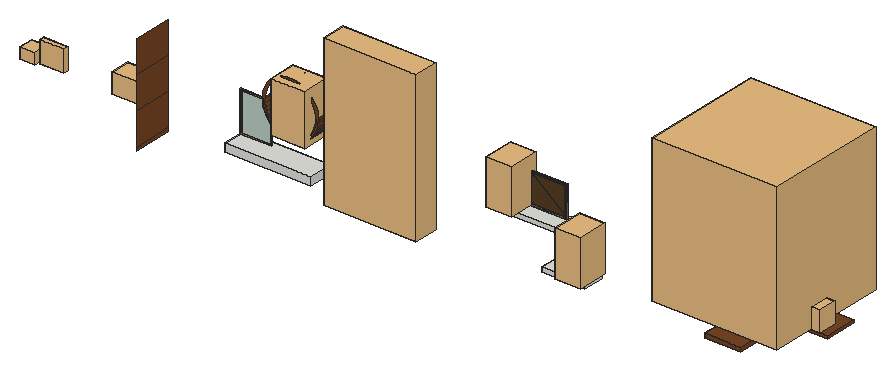
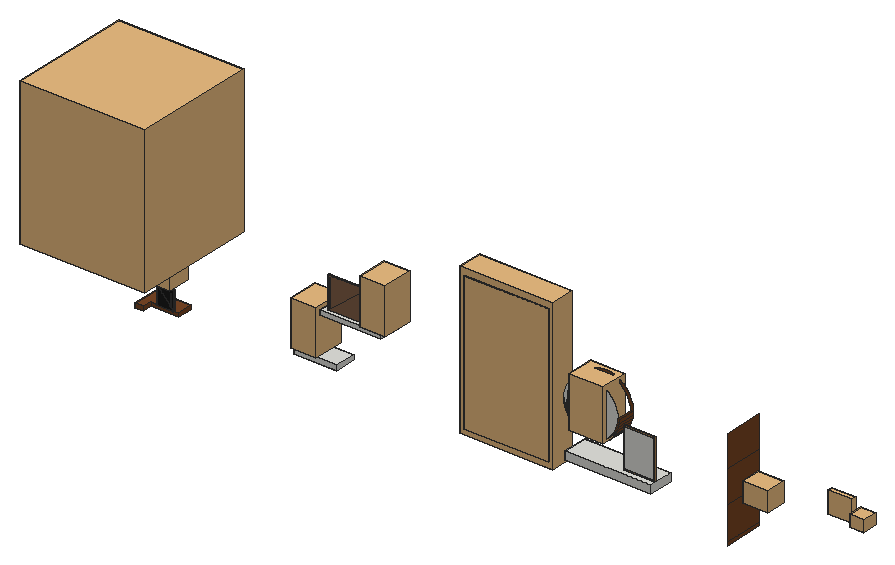
# SketchUp Ruby script. Lengths in inches.
U = 1.inch
M = Sketchup.active_model
def pt(a) = Geom::Point3d.new(a.map { |v| v * U })
def face(e, loops, mat)
  f = e.add_face(loops[0].map { |a| pt(a) })
  loops[1..].each { |l| e.add_face(l.map { |a| pt(a) }).erase! }
  f.material = f.back_material = mat if mat
  f
end
# faces: each face lists its corners as indices into pts; further lists are holes
def faces(e, pts, list, mat = nil) = list.each { |f| face(e, (f[0].is_a?(Array) ? f : [f]).map { |l| l.map { |i| pts[i] } }, mat) }
# xy, xz, yz: faces in a plane at the given z, y or x. An outline is a flat list of corners, or four numbers for a rectangle; further outlines are holes
def ring(l) = l.size == 4 ? [[l[0], l[1]], [l[2], l[1]], [l[2], l[3]], [l[0], l[3]]] : l.each_slice(2).to_a
def flat(e, list, mat, &to3) = list.each { |f| face(e, (f[0].is_a?(Array) ? f : [f]).map { |l| ring(l).map { |u, v| to3.(u, v) } }, mat) }
def xy(e, z, list, mat = nil) = flat(e, list, mat) { |x, y| [x, y, z] }
def xz(e, y, list, mat = nil) = flat(e, list, mat) { |x, z| [x, y, z] }
def yz(e, x, list, mat = nil) = flat(e, list, mat) { |y, z| [x, y, z] }
def lines(e, pts, list) = list.each { |a, b| e.add_line(pt(pts[a]), pt(pts[b])) }
# prism: a flat outline (further loops are holes) pulled along v
def prism(e, loops, v, mat = nil)
  f = face(e, loops, mat); d = Geom::Vector3d.new(v.map { |x| x * U })
  f.pushpull(f.normal.samedirection?(d) ? d.length : -d.length)
end
def box(e, o, s, mat = nil) = prism(e, [[o, [o[0] + s[0], o[1], o[2]], [o[0] + s[0], o[1] + s[1], o[2]], [o[0], o[1] + s[1], o[2]]]], [0, 0, s[2]], mat)
def at(x, y, z, deg = 0) = Geom::Transformation.translation(pt([x, y, z])) * Geom::Transformation.rotation(ORIGIN, Z_AXIS, deg.degrees)
def axes(o, x, y, z) = Geom::Transformation.new([*x, 0, *y, 0, *z, 0, *pt(o).to_a, 1])
def part(name) = M.definitions.add(name)
# library, detail: a bought-in or finely detailed component or shape, given as its bounding box
def library(name, o, s) = part(name).tap { |d| box(d.entities, o, s) }
def detail(e, o, s) = box(e.add_group.entities, o, s)
def put(e, d, t, mat = nil) = e.add_instance(d, t).tap { |i| i.material = mat if mat }
def group(e, t, mat = nil) = e.add_group.tap { |g| g.transformation = t; g.material = mat if mat }.entities
root = M.entities
M.materials.add("F5").color = [187, 207, 196]
M.materials.add("Material~40").color = [127, 90, 70]
M.materials.add("Material~42").color = [132, 97, 74]
M.materials.add("Material~43").color = [85, 62, 36]
M.materials.add("Material~5").color = [255, 255, 255]
M.materials.add("Material~67").color = [134, 108, 92]
M.materials.add("Material~8").color = [30, 30, 30]
M.materials.add("Querkus Oak Naturel Adagio _ Architonic1").color = [173, 130, 81]
M.materials.add("[Wood Veneer 01]").color = [120, 70, 37]
M.materials.add("mediterranean-hardwood-flooring").color = [114, 82, 60]
c1 = library("books",[6.19,-1.3125,-0.22],[15.35,11.9,12.07])
c2 = library("_CAPIM_DOS_PAMPAS_JULIAAIRES.3D",[-3.51,-2.78,-196.14],[35.86,35.18,43.25])
c3 = library("Group\#3",[-0.5,-0.5,0],[51.2,7,83.38])
c4 = library("Group\#408",[-8.45,0,0],[43.88,32.57,13.98])
c5 = library("Group\#388",[0,403.15,0],[76.9,397.92,354.24])
c6 = library("Group\#612",[-1.11,-0.87,0],[7.59,7.6,5.76])
c7 = library("Potted croton",[2.12,-0.7,0],[25.93,26.45,60.75])
c8 = part("3DGeom~28_Defintion")
xy(c8.entities,0,[[-149.11,-1058.59,-149.11,-248.91,850.89,-248.91],[-149.11,-1058.59,850.89,-248.91,850.89,-1058.59]])
xy(c8.entities,7.8,[[-108.07,-1017.55,809.85,-1017.55,809.85,-289.57],[-108.07,-1017.55,809.85,-289.57,-108.07,-289.57]])
xz(c8.entities,-1058.59,[[-149.11,0,-147.23,31.11,-149.11,29.78],[-149.11,0,850.89,0,-147.23,31.11],[850.89,0,849.01,31.11,-147.23,31.11],[850.89,0,850.89,29.78,849.01,31.11],[-149.11,27.12,-149.11,29.78,-147.23,31.11],
  [850.89,27.12,849.01,31.11,850.89,29.78]])
xz(c8.entities,-1017.55,[[-108.07,7.8,-106.19,19.93,809.85,7.8],[-108.07,7.8,-108.07,18.6,-106.19,19.93],[809.85,7.8,-106.19,19.93,809.85,18.6],[-108.07,15.94,-106.19,19.93,-108.07,18.6],[809.85,15.94,809.85,18.6,807.97,19.93],
  [809.85,18.6,-106.19,19.93,807.97,19.93]])
xz(c8.entities,-289.57,[[-108.07,7.8,807.97,19.93,-108.07,18.6],[-108.07,7.8,809.85,7.8,807.97,19.93],[809.85,7.8,809.85,18.6,807.97,19.93],[-108.07,15.94,-108.07,18.6,-106.19,19.93],[809.85,15.94,807.97,19.93,809.85,18.6],
  [-108.07,18.6,807.97,19.93,-106.19,19.93]])
xz(c8.entities,-248.91,[[-149.11,0,-147.23,31.11,849.01,31.11],[-149.11,0,-149.11,29.78,-147.23,31.11],[-149.11,0,849.01,31.11,850.89,0],[850.89,0,849.01,31.11,850.89,29.78],[-149.11,27.12,-147.23,31.11,-149.11,29.78],
  [850.89,27.12,850.89,29.78,849.01,31.11]])
yz(c8.entities,-149.11,[[-1058.59,27.12,-1056.71,31.11,-1058.59,29.78],[-248.91,27.12,-248.91,29.78,-250.79,31.11]])
yz(c8.entities,-108.07,[[-1017.55,15.94,-1017.55,18.6,-1015.67,19.93],[-289.57,15.94,-291.45,19.93,-289.57,18.6]])
yz(c8.entities,809.85,[[-1017.55,15.94,-1015.67,19.93,-1017.55,18.6],[-289.57,15.94,-289.57,18.6,-291.45,19.93]])
yz(c8.entities,850.89,[[-1058.59,27.12,-1058.59,29.78,-1056.71,31.11],[-248.91,27.12,-250.79,31.11,-248.91,29.78]])
p = [[-149.11,-1056.71,31.11],[-149.11,-1058.59,27.12],[-108.07,-1017.55,15.94],[-106.19,-1017.55,19.93],[-108.07,-1017.55,15.94],[-149.11,-1058.59,27.12],
  [809.85,-1017.55,15.94],[807.97,-1017.55,19.93],[849.01,-1058.59,31.11],[850.89,-1058.59,27.12],[809.85,-1015.67,19.93],[809.85,-1017.55,15.94],
  [850.89,-1058.59,27.12],[-108.07,-1015.67,19.93],[-108.07,-291.45,19.93],[-108.07,-289.57,15.94],[-149.11,-248.91,27.12],[809.85,-289.57,15.94],
  [809.85,-291.45,19.93],[850.89,-250.79,31.11],[-147.23,-248.91,31.11],[-149.11,-248.91,27.12],[-108.07,-289.57,15.94],[-106.19,-289.57,19.93],
  [807.97,-289.57,19.93],[809.85,-289.57,15.94],[850.89,-248.91,27.12],[850.89,-248.91,27.12],[-147.23,-1058.59,31.11],[-106.19,-1017.55,19.93],
  [-147.23,-1058.59,31.11],[849.01,-1058.59,31.11],[807.97,-1017.55,19.93],[850.89,-1056.71,31.11],[-149.11,-250.79,31.11],[807.97,-289.57,19.93],
  [849.01,-248.91,31.11],[-147.23,-248.91,31.11],[-106.19,-289.57,19.93],[849.01,-248.91,31.11]]
faces(c8.entities,p,[[0,1,2],[3,4,5],[6,7,8],[8,9,6],[10,11,12],[2,13,0],[14,15,16],[17,18,19],
  [20,21,22],[22,23,20],[24,25,26],[19,27,17],[5,28,3],[29,30,31],[31,32,29],[12,33,10],
  [16,34,14],[35,36,37],[37,38,35],[26,39,24]])
c9 = part("Group116\#1")
put(c9.entities,c8,axes([4.57,-0.61,76.9375],[-0.0234,0,0],[0,0,0.0234],[0,-0.02306,0]),"Material~42")
c10 = part("Group115\#1")
put(c10.entities,c9,at(0,0,0))
c11 = part("3DGeom~29_Defintion")
xy(c11.entities,0,[[-117.73,-1108.53,-113.39,-1104.19,877.92,-1104.19],[-117.73,-1108.53,-117.73,-315.47,-113.39,-1104.19],[-117.73,-1108.53,877.92,-1104.19,882.27,-1108.53],[882.27,-1108.53,877.92,-1104.19,877.92,-319.81],[882.27,-1108.53,877.92,-319.81,882.27,-315.47],
  [-113.39,-1104.19,-117.73,-315.47,-113.39,-319.81],[-113.39,-319.81,-117.73,-315.47,882.27,-315.47],[-113.39,-319.81,882.27,-315.47,877.92,-319.81]])
xy(c11.entities,14.47,[[-117.73,-1108.53,-113.39,-1104.19,-117.73,-315.47],[-117.73,-1108.53,877.92,-1104.19,-113.39,-1104.19],[-117.73,-1108.53,882.27,-1108.53,877.92,-1104.19],[882.27,-1108.53,877.92,-319.81,877.92,-1104.19],[882.27,-1108.53,882.27,-315.47,877.92,-319.81],
  [-113.39,-1104.19,-113.39,-319.81,-117.73,-315.47],[-113.39,-319.81,882.27,-315.47,-117.73,-315.47],[-113.39,-319.81,877.92,-319.81,882.27,-315.47]])
xz(c11.entities,-1108.53,[[-117.73,0,882.27,0,882.27,14.47],[-117.73,0,882.27,14.47,-117.73,14.47]])
xz(c11.entities,-1104.19,[[-113.39,0,-113.39,14.47,877.92,0],[877.92,0,-113.39,14.47,877.92,14.47]])
xz(c11.entities,-319.81,[[-113.39,0,877.92,0,877.92,14.47],[-113.39,0,877.92,14.47,-113.39,14.47]])
xz(c11.entities,-315.47,[[-117.73,0,-117.73,14.47,882.27,0],[882.27,0,-117.73,14.47,882.27,14.47]])
yz(c11.entities,-117.73,[[-1108.53,0,-1108.53,14.47,-315.47,0],[-315.47,0,-1108.53,14.47,-315.47,14.47]])
yz(c11.entities,-113.39,[[-1104.19,0,-319.81,0,-319.81,14.47],[-1104.19,0,-319.81,14.47,-1104.19,14.47]])
yz(c11.entities,877.92,[[-1104.19,0,-1104.19,14.47,-319.81,0],[-319.81,0,-1104.19,14.47,-319.81,14.47]])
yz(c11.entities,882.27,[[-1108.53,0,-315.47,0,-315.47,14.47],[-1108.53,0,-315.47,14.47,-1108.53,14.47]])
c12 = part("Group118\#1")
put(c12.entities,c11,axes([4.57,-0.79,76.9375],[-0.02148,0,0],[0,0,0.02148],[0,-0.02117,0]),"Material~40")
c13 = part("Group117\#1")
put(c13.entities,c12,at(0,0,0))
c14 = part("3DGeom~27_Defintion")
yz(c14.entities,-149.11,[[-1058.59,0,-1056.71,31.11,-250.79,31.11],[-1058.59,0,-1058.59,29.78,-1056.71,31.11],[-1058.59,0,-250.79,31.11,-248.91,0],[-248.91,0,-250.79,31.11,-248.91,29.78]])
yz(c14.entities,-108.07,[[-1017.55,7.8,-289.57,7.8,-291.45,19.93],[-1017.55,7.8,-291.45,19.93,-1017.55,18.6],[-289.57,7.8,-289.57,18.6,-291.45,19.93],[-1017.55,18.6,-291.45,19.93,-1015.67,19.93]])
yz(c14.entities,809.85,[[-1017.55,7.8,-1015.67,19.93,-289.57,7.8],[-1017.55,7.8,-1017.55,18.6,-1015.67,19.93],[-289.57,7.8,-1015.67,19.93,-289.57,18.6],[-289.57,18.6,-1015.67,19.93,-291.45,19.93]])
yz(c14.entities,850.89,[[-1058.59,0,-1056.71,31.11,-1058.59,29.78],[-1058.59,0,-248.91,0,-1056.71,31.11],[-248.91,0,-250.79,31.11,-1056.71,31.11],[-248.91,0,-248.91,29.78,-250.79,31.11]])
p = [[-108.07,-291.45,19.93],[-149.11,-250.79,31.11],[-149.11,-1056.71,31.11],[-108.07,-1015.67,19.93],[809.85,-1015.67,19.93],[850.89,-1056.71,31.11],
  [850.89,-250.79,31.11],[809.85,-291.45,19.93]]
faces(c14.entities,p,[[0,1,2],[2,3,0],[4,5,6],[6,7,4]])
c15 = part("Group114\#1")
put(c15.entities,c14,axes([4.57,-0.61,76.9375],[-0.0234,0,0],[0,0,0.0234],[0,-0.02306,0]),"Material~42")
c16 = part("Group113\#2")
put(c16.entities,c15,at(0,0,0))
c17 = part("3DGeom~26_Defintion")
xy(c17.entities,0,[[-114.39,-1113.87,-114.39,-322.61,885.61,-322.61],[-114.39,-1113.87,885.61,-322.61,885.61,-1113.87]],"Material~43")
xy(c17.entities,1.46,[[-114.39,-1113.87,885.61,-1113.87,885.61,-322.61],[-114.39,-1113.87,885.61,-322.61,-114.39,-322.61]],"Material~43")
xz(c17.entities,-1113.87,[[-114.39,0,885.61,0,885.61,1.46],[-114.39,0,885.61,1.46,-114.39,1.46]])
xz(c17.entities,-322.61,[[-114.39,0,-114.39,1.46,885.61,0],[885.61,0,-114.39,1.46,885.61,1.46]])
yz(c17.entities,-114.39,[[-1113.87,0,-1113.87,1.46,-322.61,0],[-322.61,0,-1113.87,1.46,-322.61,1.46]])
yz(c17.entities,885.61,[[-1113.87,0,-322.61,0,-322.61,1.46],[-1113.87,0,-322.61,1.46,-1113.87,1.46]])
c18 = part("Group112\#2")
put(c18.entities,c17,axes([4.57,-0.8,76.9375],[-0.02129,0,0],[0,0,0.02129],[0,-0.02099,0]),"Material~43")
c19 = part("Group111\#2")
put(c19.entities,c18,at(0,0,0))
c20 = part("3DGeom~47_Defintion\#2")
xy(c20.entities,79.8821,[[-809.2892,798.889,52.5331,798.8892,100.4623,798.889]])
xy(c20.entities,79.8826,[[-857.2183,-201.1106,-809.2891,-153.181,-857.2181,-153.1814],[-857.2183,-201.1106,-809.2891,-201.1106,-809.2891,-153.181],[-809.2891,-201.1106,52.5332,-153.1813,-809.2891,-153.181]])
xz(c20.entities,-201.1106,[[-857.2183,0.0003,-809.2891,79.8826,-857.2183,79.8826]])
xz(c20.entities,798.889,[[-857.2182,-0.0002,-809.2892,79.8821,100.4623,79.8821],[-857.2182,-0.0002,-857.2182,79.8821,-809.2892,79.8821]])
yz(c20.entities,100.4624,[[-201.1107,0.0003,-153.1813,79.8826,-201.1107,79.8825]])
p = [[-857.2182,798.889,-0.0002],[-857.2183,-201.1106,0.0003],[-857.2183,-201.1106,79.8826],[-857.2181,-153.1814,79.8826],[-857.2183,-201.1106,0.0003],[100.4624,-201.1107,0.0003],
  [100.4624,-201.1107,79.8825],[52.5332,-201.1104,79.8825],[-809.2891,-201.1106,79.8826],[100.4623,798.8893,-0.0002],[100.4624,-201.1107,0.0003],[-857.2183,-201.1106,0.0003],
  [-857.2182,798.889,-0.0002],[100.4624,-201.1107,0.0003],[100.4623,798.8893,-0.0002],[100.4623,798.889,79.8821],[100.462,750.9601,79.882],[100.4624,-153.1813,79.8826],
  [-857.2184,750.9597,79.882],[-857.2182,798.889,79.8821],[-857.2182,798.889,-0.0002],[100.4623,798.889,79.8821],[100.4623,798.8893,-0.0002],[-809.2891,-153.1812,31.9533],
  [-809.2892,750.96,31.9527],[-809.2892,750.96,79.882],[-809.2891,-153.181,79.8826],[52.5332,-153.1813,31.9532],[-809.2891,-153.1812,31.9533],[-809.2891,-153.181,79.8826],
  [-809.2891,-153.181,79.8826],[52.5332,-153.1813,79.8826],[52.5332,-153.1813,31.9532],[52.5331,750.9599,31.9527],[52.5332,-153.1813,31.9532],[52.5332,-153.1813,79.8826],
  [52.5331,750.9601,79.882],[-809.2892,750.96,31.9527],[52.5331,750.9599,31.9527],[52.5331,750.9601,79.882],[52.5331,750.9601,79.882],[-809.2892,750.96,79.882],
  [-809.2892,750.96,31.9527],[52.5332,-201.1104,79.8825],[52.5332,-153.1813,79.8826],[-809.2891,-201.1106,79.8826],[100.4624,-153.1813,79.8826],[100.4624,-201.1107,79.8825],
  [-857.2181,-153.1814,79.8826],[-809.2891,-153.181,79.8826],[-809.2892,750.96,79.882],[-857.2184,750.9597,79.882],[52.5331,750.9601,79.882],[100.462,750.9601,79.882],
  [-809.2892,798.889,79.8821],[-857.2182,798.889,79.8821],[52.5331,798.8892,79.8821],[100.4623,798.889,79.8821]]
faces(c20.entities,p,[[0,1,2],[0,2,3],[4,5,6],[4,6,7],[4,7,8],[9,10,11],[9,11,12],[13,14,15],
  [13,15,16],[13,16,17],[0,3,18],[0,18,19],[20,21,22],[23,24,25],[25,26,23],[27,28,29],
  [30,31,32],[33,34,35],[35,36,33],[37,38,39],[40,41,42],[43,44,45],[46,44,43],[47,46,43],
  [48,49,50],[48,50,51],[52,44,53],[53,44,46],[51,50,54],[55,51,54],[54,50,56],[56,50,52],
  [56,52,57],[57,52,53]])
c21 = part("Group152\#2")
put(c21.entities,c20,axes([-5.78,-0.65,75.89],[0.01115,0,0],[0,0,0.01115],[0,-0.01115,0]),"Material~8")
c22 = part("3DGeom~48_Defintion\#1")
xy(c22.entities,35.34,[[-895.09,-169.42,-774.33,-48.66,-895.09,830.58],[-895.09,-169.42,58.1,-169.42,-774.33,-48.66],[58.1,-169.42,-62.66,-48.66,-774.33,-48.66],[58.1,-169.42,-62.66,709.82,-62.66,-48.66],[58.1,-169.42,58.1,830.58,-62.66,709.82],
  [-774.33,-48.66,-774.33,709.82,-895.09,830.58],[-774.33,709.82,58.1,830.58,-895.09,830.58],[-774.33,709.82,-62.66,709.82,58.1,830.58]])
xz(c22.entities,-48.66,[[-62.66,17.67,-774.33,35.34,-62.66,35.34],[-774.33,17.67,-774.33,35.34,-62.66,17.67]])
xz(c22.entities,709.82,[[-774.33,17.67,-62.66,17.67,-62.66,35.34],[-774.33,17.67,-62.66,35.34,-774.33,35.34]])
yz(c22.entities,-774.33,[[-48.66,17.67,709.82,17.67,709.82,35.34],[-48.66,17.67,709.82,35.34,-48.66,35.34]])
yz(c22.entities,-62.66,[[-48.66,17.67,-48.66,35.34,709.82,17.67],[709.82,17.67,-48.66,35.34,709.82,35.34]])
c23 = part("Group153\#2")
put(c23.entities,c22,axes([-5.78,-0.65,75.89],[0.01008,0,0],[0,0,0.01008],[0,-0.01008,0]),"Material~5")
c24 = part("3DGeom~49_Defintion\#1")
xy(c24.entities,23.3,[[-1020.9,-64.15,-82.61,-64.15,-82.61,935.85],[-1020.9,-64.15,-82.61,935.85,-1020.9,935.85]],"Material~67")
c25 = part("Group154\#2")
put(c25.entities,c24,axes([-5.78,-0.65,75.89],[0.00765,0,0],[0,0,0.00765],[0,-0.00765,0]),"Material~67")
c26 = part("Group151\#2")
put(c26.entities,c21,at(0,0,0))
put(c26.entities,c23,at(0,0,0))
put(c26.entities,c25,at(0,0,0))
c27 = library("Potted foliage plant",[-34.87,-29.84,0],[109.95,108.62,128.4])
c28 = library("Architecture and design books\#1",[9.67,-0.02,0],[20.02,11.1,12.25])
box(root,[153.34,11.47,49.37],[52,15,5])
box(root,[317.6,12.47,75.14],[37.4,13,2.87])
box(root,[343.26,13.97,49.81],[26.4,13,2.87])
xy(root,66,[[188.91,16.47,189.91,26.47]],"[Wood Veneer 01]")
xy(root,67.39,[[187.93,16.47,189.89,26.47]],"[Wood Veneer 01]")
xy(root,74.65,[[468.11,13.47,517.11,33.47]],"[Wood Veneer 01]")
xy(root,76.65,[[468.11,13.47,517.11,33.47]],"[Wood Veneer 01]")
xz(root,13.47,[[468.11,74.65,517.11,76.65]],"[Wood Veneer 01]")
xz(root,16.47,[[[187.84,66,189.98,66,191.91,66.24,192.1,66.27,192.91,66.48,194.16,66.8,194.91,67.09,195.91,67.49,196.15,67.58,197.91,68.55,198.02,68.61,198.91,69.26,199.75,69.87,200.91,70.96,201.3,71.33,202.66,72.97,203.81,74.78,204.72,76.71,205.375,78.74,205.78,80.84,205.91,82.97,205.78,85.1,205.375,87.19,204.72,89.22,203.81,91.16,202.66,92.96,201.3,94.6,200.91,94.97,199.75,96.0625,198.91,96.67,198.02,97.32,197.91,97.38,196.15,98.35,195.91,98.44,194.91,98.84,194.16,99.13,192.91,99.46,192.1,99.66,191.91,99.6875,189.98,99.93,187.84,99.93,186.91,99.8125,185.91,99.6875,185.72,99.66,183.91,99.2,183.66,99.13,182.91,98.84,181.67,98.35,180.91,97.93,179.91,97.38,179.8,97.32,178.07,96.0625,177.91,95.91,176.52,94.6,175.16,92.96,174.01,91.16,173.1,89.22,172.44,87.19,172.04,85.1,171.91,82.97,172.04,80.84,172.44,78.74,173.1,76.71,174.01,74.78,175.16,72.97,176.52,71.33,177.91,70.02,178.07,69.87,179.8,68.61,179.91,68.55,180.91,68,181.67,67.58,182.91,67.09,183.66,66.8,183.91,66.73,185.72,66.27,185.91,66.24,186.91,66.12],[187.93,67.39,187.08,67.49,186.08,67.62,185.98,67.63,184.25,68.08,184.09,68.12,183.42,68.38,182.26,68.84,181.58,69.22,180.58,69.77,180.55,69.79,178.96,70.9375,178.86,71.03,177.53,72.28,176.28,73.79,175.23,75.45,174.4,77.22,173.79,79.08,173.42,81.01,173.3,82.97,173.42,84.92,173.79,86.85,174.4,88.71,175.23,90.49,176.28,92.14,177.53,93.65,178.86,94.9,178.96,94.99,180.55,96.15,180.58,96.16,181.58,96.71,182.26,97.09,183.42,97.55,184.09,97.8125,184.25,97.85,185.98,98.3,187.08,98.4375,187.93,98.54,189.89,98.54,191.74,98.3125,191.83,98.3,192.56,98.11,193.73,97.8125,194.4,97.55,195.4,97.15,195.56,97.09,197.24,96.16,197.27,96.15,198.09,95.55,198.86,94.99,199.96,93.96,200.29,93.65,201.54,92.14,202.59,90.49,203.42,88.71,204.03,86.85,204.4,84.92,204.52,82.97,204.4,81.01,204.03,79.08,203.42,77.22,202.59,75.45,201.54,73.79,200.29,72.28,199.96,71.97,198.86,70.9375,198.09,70.38,197.27,69.79,197.24,69.77,195.56,68.84,195.4,68.78,194.4,68.38,193.73,68.12,192.56,67.82,191.83,67.63,191.74,67.62,189.89,67.39]]],"[Wood Veneer 01]")
xz(root,26.47,[[187.93,67.39,189.89,67.39,191.74,67.62,191.83,67.63,192.56,67.82,193.73,68.12,194.4,68.38,195.4,68.78,195.56,68.84,197.24,69.77,197.27,69.79,198.09,70.38,198.86,70.9375,199.96,71.97,200.29,72.28,200.91,73.03,201.54,73.79,202.59,75.45,203.42,77.22,204.03,79.08,204.4,81.01,204.52,82.97,204.4,84.92,204.03,86.85,203.42,88.71,202.59,90.49,201.54,92.14,200.91,92.9,200.29,93.65,199.96,93.96,198.86,94.99,198.09,95.55,197.27,96.15,197.24,96.16,195.56,97.09,195.4,97.15,194.4,97.55,193.73,97.8125,192.56,98.11,191.83,98.3,191.74,98.3125,189.89,98.54,187.93,98.54,187.08,98.4375,185.98,98.3,184.25,97.85,184.09,97.8125,183.42,97.55,182.26,97.09,181.58,96.71,180.58,96.16,180.55,96.15,178.96,94.99,178.86,94.9,177.53,93.65,176.28,92.14,175.23,90.49,174.4,88.71,173.79,86.85,173.42,84.92,173.3,82.97,173.42,81.01,173.79,79.08,174.4,77.22,175.23,75.45,176.28,73.79,177.53,72.28,178.86,71.03,178.96,70.9375,180.55,69.79,180.58,69.77,181.58,69.22,182.26,68.84,183.42,68.38,184.09,68.12,184.25,68.08,185.98,67.63,186.08,67.62,187.08,67.49],[200.91,70.96,201.3,71.33,202.66,72.97,203.81,74.78,204.72,76.71,205.375,78.74,205.78,80.84,205.91,82.97,205.78,85.1,205.375,87.19,204.72,89.22,203.81,91.16,202.66,92.96,201.3,94.6,200.91,94.97,200.91,92.9,201.54,92.14,202.59,90.49,203.42,88.71,204.03,86.85,204.4,84.92,204.52,82.97,204.4,81.01,204.03,79.08,203.42,77.22,202.59,75.45,201.54,73.79,200.91,73.03]])
xz(root,33.47,[[468.11,74.65,517.11,76.65]])
yz(root,106.84,[[2.47,37.59,26.47,39.59],[2.47,39.59,26.47,59.52],[2.47,59.52,26.47,78.95],[2.47,78.95,26.47,98.39]],"[Wood Veneer 01]")
yz(root,468.11,[[13.47,74.65,33.47,76.65]],"[Wood Veneer 01]")
yz(root,517.11,[[13.47,74.65,33.47,76.65]],"[Wood Veneer 01]")
p = [[185.91,26.47,66.24],[186.91,26.47,66.12],[186.91,16.47,66.12],[185.91,16.47,66.24],[185.91,25.47,66.24],[185.72,25.47,66.27],
  [185.72,16.47,66.27],[191.91,26.47,66.24],[192.1,26.47,66.27],[192.1,16.47,66.27],[191.91,16.47,66.24],[183.91,25.47,66.73],
  [183.91,16.47,66.73],[192.91,26.47,66.48],[192.91,16.47,66.48],[183.66,26.47,66.8],[183.91,26.47,66.73],[183.66,16.47,66.8],
  [182.91,26.47,67.09],[182.91,16.47,67.09],[194.91,26.47,67.09],[195.91,26.47,67.49],[195.91,16.47,67.49],[194.91,16.47,67.09],
  [187.93,26.47,67.39],[187.08,26.47,67.49],[186.08,26.47,67.62],[185.98,26.47,67.63],[185.98,16.47,67.63],[186.08,16.47,67.62],
  [187.08,16.47,67.49],[187.93,16.47,67.39],[191.83,26.47,67.63],[191.74,26.47,67.62],[189.89,26.47,67.39],[189.89,16.47,67.39],
  [191.74,16.47,67.62],[191.83,16.47,67.63],[184.25,26.47,68.08],[184.09,26.47,68.12],[184.09,16.47,68.12],[184.25,16.47,68.08],
  [193.73,26.47,68.12],[192.56,26.47,67.82],[192.56,16.47,67.82],[193.73,16.47,68.12],[179.91,26.47,68.55],[180.91,26.47,68],
  [180.91,16.47,68],[179.91,16.47,68.55],[183.42,26.47,68.38],[182.26,26.47,68.84],[182.26,16.47,68.84],[183.42,16.47,68.38],
  [195.4,26.47,68.78],[194.4,26.47,68.38],[194.4,16.47,68.38],[195.4,16.47,68.78],[195.56,16.47,68.84],[195.56,26.47,68.84],
  [197.91,26.47,68.55],[198.02,26.47,68.61],[198.02,16.47,68.61],[197.91,16.47,68.55],[198.91,26.47,69.26],[198.91,16.47,69.26],
  [181.58,26.47,69.22],[180.58,26.47,69.77],[180.55,26.47,69.79],[180.55,16.47,69.79],[180.58,16.47,69.77],[181.58,16.47,69.22],
  [197.27,26.47,69.79],[197.24,26.47,69.77],[197.24,16.47,69.77],[197.27,16.47,69.79],[178.96,26.47,70.9375],[178.96,16.47,70.9375],
  [198.86,26.47,70.9375],[198.09,26.47,70.38],[198.09,16.47,70.38],[198.86,16.47,70.9375],[176.52,26.47,71.33],[177.91,26.47,70.02],
  [177.91,16.47,70.02],[176.52,16.47,71.33],[178.86,26.47,71.03],[177.53,26.47,72.28],[177.53,16.47,72.28],[178.86,16.47,71.03],
  [200.29,26.47,72.28],[199.96,26.47,71.97],[199.96,16.47,71.97],[200.29,16.47,72.28],[200.91,16.47,70.96],[200.91,22.47,70.96],
  [201.3,22.47,71.33],[201.3,16.47,71.33],[200.91,26.47,70.96],[201.3,26.47,71.33],[175.16,26.47,72.97],[175.16,16.47,72.97],
  [202.66,22.47,72.97],[202.66,16.47,72.97],[202.66,26.47,72.97],[176.28,26.47,73.79],[176.28,16.47,73.79],[200.91,26.47,73.03],
  [201.54,16.47,73.79],[201.54,26.47,73.79],[174.01,26.47,74.78],[174.01,16.47,74.78],[203.81,22.47,74.78],[203.81,16.47,74.78],
  [203.81,26.47,74.78],[175.23,26.47,75.45],[175.23,16.47,75.45],[202.59,26.47,75.45],[202.59,16.47,75.45],[173.1,26.47,76.71],
  [173.1,16.47,76.71],[204.72,22.47,76.71],[204.72,16.47,76.71],[204.72,26.47,76.71],[174.4,26.47,77.22],[174.4,16.47,77.22],
  [203.42,26.47,77.22],[203.42,16.47,77.22],[172.44,26.47,78.74],[172.44,16.47,78.74],[205.375,22.47,78.74],[205.375,16.47,78.74],
  [205.375,26.47,78.74],[173.79,26.47,79.08],[173.79,16.47,79.08],[204.03,26.47,79.08],[204.03,16.47,79.08],[172.04,26.47,80.84],
  [172.04,16.47,80.84],[205.78,22.47,80.84],[205.78,16.47,80.84],[205.78,26.47,80.84],[173.42,26.47,81.01],[173.42,16.47,81.01],
  [204.4,26.47,81.01],[204.4,16.47,81.01],[171.91,26.47,82.97],[171.91,16.47,82.97],[205.91,22.47,82.97],[205.91,16.47,82.97],
  [205.91,26.47,82.97],[173.3,26.47,82.97],[173.3,16.47,82.97],[204.52,26.47,82.97],[204.52,16.47,82.97]]
faces(root,p,[[0,1,2,3,4],[7,8,9,10],[8,13,14,9],[15,16,11,12,17],[18,15,17,19],[20,21,22,23],[24,25,26,27,28,29,30,31],[32,33,34,35,36,37],
  [27,38,39,40,41,28],[42,43,32,37,44,45],[46,47,48,49],[39,50,51,52,53,40],[54,55,42,45,56,57,58,59],[60,61,62,63],[61,64,65,62],[51,66,67,68,69,70,71,52],
  [72,73,59,58,74,75],[68,76,77,69],[78,79,72,75,80,81],[82,83,84,85],[76,86,87,88,89,77],[90,91,78,81,92,93],[94,95,96,97],[100,82,85,101],
  [97,96,102,103],[87,105,106,88],[107,90,93,108,109],[110,100,101,111],[103,102,112,113],[105,115,116,106],[117,109,108,118],[119,110,111,120],
  [113,112,121,122],[115,124,125,116],[126,117,118,127],[128,119,120,129],[122,121,130,131],[124,133,134,125],[135,126,127,136],[137,128,129,138],
  [131,130,139,140],[133,142,143,134],[144,135,136,145],[146,137,138,147],[140,139,148,149],[142,151,152,143],[153,144,145,154]],"[Wood Veneer 01]")
faces(root,p,[[5,4,3,6],[11,5,6,12],[98,99,96,95],[99,104,102,96],[104,114,112,102],[114,123,121,112],[123,132,130,121],[132,141,139,130],
  [141,150,148,139]])
detail(root,[212.91,11.47,41.58],[56.38,15,90.68])
put(root,c1,at(81.29,9.47,59.52))
g1 = group(root,at(153.34,22.87,54.37))
xy(g1,0.5,[[0.5,0.3,18.5,0.6]])
xy(g1,24,[[0.5,0.3,18.5,0.6]])
xz(g1,0.3,[[0.5,0.5,18.5,24]],"F5")
xz(g1,0.6,[[0.5,0.5,18.5,24]])
yz(g1,0.5,[[0.3,0.5,0.6,24]])
yz(g1,18.5,[[0.3,0.5,0.6,24]])
g2 = group(g1,at(0,0,0),"Querkus Oak Naturel Adagio _ Architonic1")
prism(g2,[[[0,0.6,0],[0,0.6,24.5],[19,0.6,24.5],[19,0.6,0]],[[0.5,0.6,0.5],[18.5,0.6,0.5],[18.5,0.6,24],[0.5,0.6,24]]],[0,-0.6,0])
put(root,c2,axes([182.54,13.35,207.62],[0.57987,0,0],[0,0.47819,0],[0,0,0.71174]))
put(root,c3,at(215.36,20.47,45.24))
g3 = group(root,at(-274.75,49.47,15.21))
put(g3,c4,axes([718.3,-21.47,100.38],[0.4514,0.00006,0.00006],[-0.00006,0,0.4331],[0.00008,-0.61,0]))
put(g3,c5,axes([306.03,-44.43,47.61],[0,0.03672,0],[0.03672,0,0],[0,0,0.03672]))
put(g3,c6,axes([311.82,-45.82,47.61],[0,1.16847,0],[1.16847,0,0],[0,0,1.16847]))
put(root,c7,axes([329.76,27.67,78.01],[0,-0.72,0],[-0.5874,0,0],[0,0,0.45]),"mediterranean-hardwood-flooring")
put(root,c10,at(343.98,23.28,25.84))
put(root,c13,at(343.98,23.28,25.84))
put(root,c16,at(343.98,23.28,25.84))
put(root,c19,at(343.98,23.28,25.84))
put(root,c7,axes([370.37,29.27,52.68],[0,-0.72,0],[-0.5874,0,0],[0,0,0.45]),"mediterranean-hardwood-flooring")
put(root,c26,at(456.41,29.01,-25.49))
g4 = group(root,at(439.53,18.47,45.73),"[Wood Veneer 01]")
prism(g4,[[[-1,9,0],[16.02,9,0],[16.02,15,0],[21.02,15,0],[21.02,0,0],[-1,0,0]]],[0,0,2.42])
g5 = group(root,at(439.53,19.47,62.07),"[Wood Veneer 01]")
detail(g5,[0,0,0],[42.02,14,76])
put(root,c27,axes([455.5,8.08,76.65],[0.69,0,0],[0,0.69,0],[0,0,0.69]))
put(root,c28,at(482.94,13.47,76.65))
